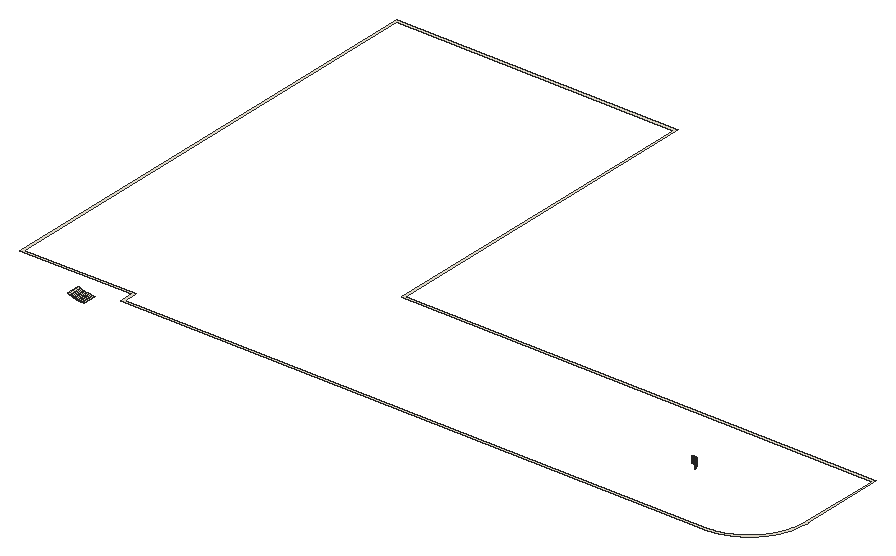
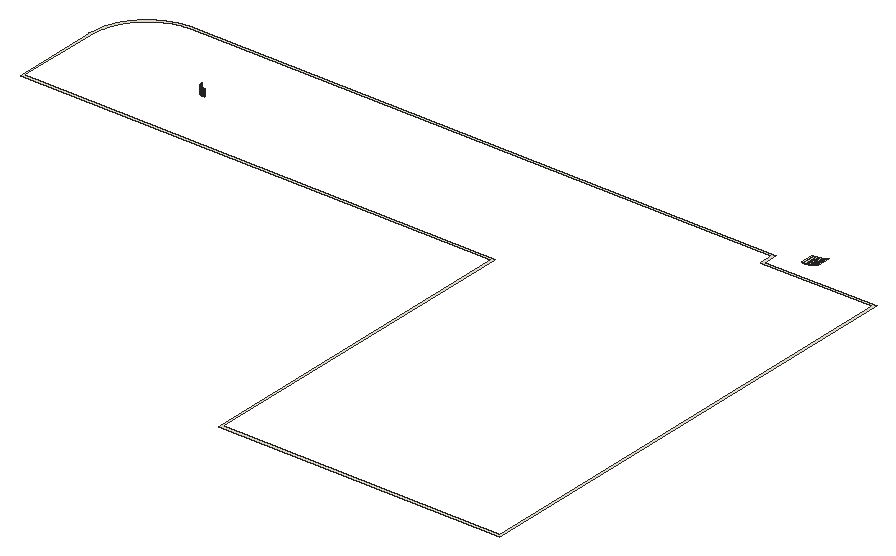
# SketchUp Ruby script. Lengths in inches.
U = 1.inch
M = Sketchup.active_model
def pt(a) = Geom::Point3d.new(a.map { |v| v * U })
def face(e, loops, mat)
  f = e.add_face(loops[0].map { |a| pt(a) })
  loops[1..].each { |l| e.add_face(l.map { |a| pt(a) }).erase! }
  f.material = f.back_material = mat if mat
  f
end
# faces: each face lists its corners as indices into pts; further lists are holes
def faces(e, pts, list, mat = nil) = list.each { |f| face(e, (f[0].is_a?(Array) ? f : [f]).map { |l| l.map { |i| pts[i] } }, mat) }
# xy, xz, yz: faces in a plane at the given z, y or x. An outline is a flat list of corners, or four numbers for a rectangle; further outlines are holes
def ring(l) = l.size == 4 ? [[l[0], l[1]], [l[2], l[1]], [l[2], l[3]], [l[0], l[3]]] : l.each_slice(2).to_a
def flat(e, list, mat, &to3) = list.each { |f| face(e, (f[0].is_a?(Array) ? f : [f]).map { |l| ring(l).map { |u, v| to3.(u, v) } }, mat) }
def xy(e, z, list, mat = nil) = flat(e, list, mat) { |x, y| [x, y, z] }
def xz(e, y, list, mat = nil) = flat(e, list, mat) { |x, z| [x, y, z] }
def yz(e, x, list, mat = nil) = flat(e, list, mat) { |y, z| [x, y, z] }
def lines(e, pts, list) = list.each { |a, b| e.add_line(pt(pts[a]), pt(pts[b])) }
# prism: a flat outline (further loops are holes) pulled along v
def prism(e, loops, v, mat = nil)
  f = face(e, loops, mat); d = Geom::Vector3d.new(v.map { |x| x * U })
  f.pushpull(f.normal.samedirection?(d) ? d.length : -d.length)
end
def box(e, o, s, mat = nil) = prism(e, [[o, [o[0] + s[0], o[1], o[2]], [o[0] + s[0], o[1] + s[1], o[2]], [o[0], o[1] + s[1], o[2]]]], [0, 0, s[2]], mat)
def at(x, y, z, deg = 0) = Geom::Transformation.translation(pt([x, y, z])) * Geom::Transformation.rotation(ORIGIN, Z_AXIS, deg.degrees)
def axes(o, x, y, z) = Geom::Transformation.new([*x, 0, *y, 0, *z, 0, *pt(o).to_a, 1])
def part(name) = M.definitions.add(name)
# library, detail: a bought-in or finely detailed component or shape, given as its bounding box
def library(name, o, s) = part(name).tap { |d| box(d.entities, o, s) }
def detail(e, o, s) = box(e.add_group.entities, o, s)
def put(e, d, t, mat = nil) = e.add_instance(d, t).tap { |i| i.material = mat if mat }
def group(e, t, mat = nil) = e.add_group.tap { |g| g.transformation = t; g.material = mat if mat }.entities
root = M.entities
M.materials.add("0027 AP L140 CRUSHED ICE").color = [241, 233, 217]
xy(root,120.5,[[[78,225,78,231,27,231,27,447,156,447,156,291,372,291,372,251.72,371.99,251.43,371.99,251.15,371.98,250.87,371.96,250.59,371.95,250.3,371.91,249.74,371.79,248.62,371.67,247.78,371.47,246.66,371.41,246.39,371.29,245.83,371.15,245.29,371.08,245.01,371.01,244.74,370.85,244.2,370.76,243.93,370.68,243.66,370.5,243.12,370.4,242.85,370.31,242.59,370.21,242.32,370.1,242.0625,370,241.8,369.67,241.02,369.43,240.5,369.31,240.25,369.18,239.99,369.06,239.74,368.8,239.24,368.66,238.99,368.52,238.75,368.38,238.5,368.24,238.26,368.09,238.01,367.95,237.77,367.8,237.53,367.64,237.29,367.49,237.06,367.33,236.82,367.01,236.36,366.84,236.13,366.68,235.9,366.51,235.68,366.33,235.45,366.16,235.23,365.62,234.57,365.4375,234.36,365.25,234.14,365.06,233.93,364.875,233.72,364.68,233.52,364.49,233.3125,364.29,233.11,363.89,232.71,363.6875,232.51,363.48,232.32,363.28,232.125,363.07,231.94,362.86,231.75,362.64,231.5625,362.43,231.38,361.77,230.84,361.55,230.67,361.32,230.49,361.1,230.32,360.87,230.16,360.64,229.99,360.18,229.67,359.94,229.51,359.71,229.36,359.47,229.2,359.23,229.05,358.99,228.91,358.74,228.76,358.5,228.62,358.25,228.48,358.01,228.34,357.76,228.2,357.26,227.94,357.01,227.82,356.75,227.69,356.5,227.57,355.98,227.33,355.2,227,354.9375,226.9,354.68,226.79,354.41,226.69,354.15,226.6,353.88,226.5,353.34,226.32,353.07,226.24,352.8,226.15,352.26,225.99,351.99,225.92,351.71,225.85,351.17,225.71,350.61,225.59,350.34,225.53,349.22,225.33,348.38,225.21,347.26,225.09,346.7,225.05,346.41,225.04,346.13,225.02,345.85,225.01,345.57,225.01,345.28,225],[79,226,345.27,226,345.54,226.01,345.82,226.01,346.09,226.02,346.36,226.04,346.63,226.05,346.9,226.07,347.18,226.09,347.45,226.12,347.72,226.14,347.99,226.17,348.26,226.21,348.53,226.24,349.34,226.36,349.6,226.41,350.14,226.51,350.41,226.57,350.67,226.625,350.9375,226.6875,351.2,226.75,351.47,226.82,352.25,227.03,352.51,227.11,352.78,227.19,353.03,227.27,353.81,227.54,354.0625,227.63,354.32,227.73,354.82,227.93,355.08,228.03,355.58,228.25,355.82,228.36,356.07,228.47,356.32,228.59,356.5625,228.71,356.8,228.83,357.05,228.96,357.53,229.22,357.76,229.35,358,229.48,358.24,229.62,358.7,229.9,358.93,230.05,359.16,230.19,359.39,230.34,359.61,230.5,359.84,230.65,360.0625,230.81,360.28,230.97,360.5,231.125,360.72,231.29,360.9375,231.46,361.15,231.625,361.36,231.79,361.57,231.97,361.78,232.14,361.99,232.32,362.19,232.5,362.4,232.68,362.6,232.86,362.8,233.05,363,233.23,363.19,233.42,363.38,233.62,363.58,233.81,363.77,234,363.95,234.2,364.14,234.4,364.32,234.6,364.5,234.81,364.68,235.01,364.86,235.22,365.03,235.43,365.21,235.64,365.375,235.85,365.54,236.0625,365.71,236.28,365.875,236.5,366.03,236.72,366.19,236.9375,366.35,237.16,366.5,237.39,366.66,237.61,366.81,237.84,366.95,238.07,367.1,238.3,367.38,238.76,367.52,239,367.65,239.24,367.78,239.47,368.04,239.95,368.17,240.2,368.29,240.4375,368.41,240.68,368.53,240.93,368.64,241.18,368.75,241.42,368.97,241.92,369.07,242.18,369.27,242.68,369.37,242.9375,369.46,243.19,369.73,243.97,369.81,244.22,369.89,244.49,369.97,244.75,370.18,245.53,370.25,245.8,370.3125,246.0625,370.375,246.33,370.43,246.59,370.49,246.86,370.59,247.4,370.64,247.66,370.76,248.47,370.79,248.74,370.83,249.01,370.86,249.28,370.88,249.55,370.91,249.82,370.93,250.1,370.95,250.37,370.96,250.64,370.98,250.91,370.99,251.18,370.99,251.46,371,251.73,371,290,155,290,155,446,28,446,28,232,79,232]]],"0027 AP L140 CRUSHED ICE")
xz(root,261,[[311.84,120,311.92,123],[311.92,120,312,123],[312,120,312.08,123],[312.08,120,312.16,123]],"0027 AP L140 CRUSHED ICE")
yz(root,315,[[258,120,258.08,123],[258.08,120,258.16,123]],"0027 AP L140 CRUSHED ICE")
p = [[67.49,216,120.05],[66.99,216,120.08],[66.99,222,120.08],[67.49,222,120.05],[67.99,216,120.02],[67.99,222,120.02],
  [68.5,216,120.01],[68.5,222,120.01],[314.98,258.3125,120],[314.99,258.24,120],[314.99,258.24,123],[314.98,258.3125,123],
  [315,258.16,120],[315,258.16,123],[314.97,258.39,120],[314.97,258.39,123],[314.96,258.47,120],[314.96,258.47,123],
  [314.93,258.625,120],[314.95,258.55,120],[314.95,258.55,123],[314.93,258.625,123],[314.92,258.7,120],[314.92,258.7,123],
  [314.9,258.78,120],[314.9,258.78,123],[314.875,258.85,120],[314.875,258.85,123],[314.83,259,120],[314.85,258.93,120],
  [314.85,258.93,123],[314.83,259,123],[314.8,259.08,120],[314.8,259.08,123],[314.74,259.22,120],[314.77,259.15,120],
  [314.77,259.15,123],[314.74,259.22,123],[314.71,259.29,120],[314.71,259.29,123],[314.67,259.36,120],[314.67,259.36,123],
  [314.6,259.5,120],[314.64,259.43,120],[314.64,259.43,123],[314.6,259.5,123],[314.56,259.57,120],[314.56,259.57,123],
  [314.47,259.7,120],[314.52,259.63,120],[314.52,259.63,123],[314.47,259.7,123],[314.43,259.76,120],[314.43,259.76,123],
  [314.33,259.89,120],[314.38,259.83,120],[314.38,259.83,123],[314.33,259.89,123],[314.23,260.01,120],[314.28,259.95,120],
  [314.28,259.95,123],[314.23,260.01,123],[314.18,260.07,120],[314.18,260.07,123],[314.07,260.18,120],[314.12,260.12,120],
  [314.12,260.12,123],[314.07,260.18,123],[313.95,260.28,120],[314.01,260.23,120],[314.01,260.23,123],[313.95,260.28,123],
  [313.83,260.38,120],[313.89,260.33,120],[313.89,260.33,123],[313.83,260.38,123],[313.7,260.47,120],[313.76,260.43,120],
  [313.76,260.43,123],[313.7,260.47,123],[313.57,260.56,120],[313.63,260.52,120],[313.63,260.52,123],[313.57,260.56,123],
  [313.36,260.67,120],[313.43,260.64,120],[313.43,260.64,123],[313.36,260.67,123],[313.5,260.6,120],[313.5,260.6,123],
  [313.15,260.77,120],[313.22,260.74,120],[313.22,260.74,123],[313.15,260.77,123],[313.29,260.71,120],[313.29,260.71,123],
  [312.93,260.85,120],[313,260.83,120],[313,260.83,123],[312.93,260.85,123],[313.08,260.8,120],[313.08,260.8,123],
  [311.3,260.92,120],[311.375,260.93,120],[311.375,260.93,123],[311.3,260.92,123],[311.45,260.95,120],[311.45,260.95,123],
  [311.53,260.96,120],[311.53,260.96,123],[312.47,260.96,120],[312.55,260.95,120],[312.55,260.95,123],[312.47,260.96,123],
  [312.625,260.93,120],[312.625,260.93,123],[312.7,260.92,120],[312.7,260.92,123],[312.78,260.9,120],[312.78,260.9,123],
  [312.85,260.875,120],[312.85,260.875,123],[311.61,260.97,120],[311.61,260.97,123],[311.6875,260.98,120],[311.6875,260.98,123],
  [311.76,260.99,120],[311.76,260.99,123],[311.84,261,120],[311.84,261,123],[312.16,261,120],[312.24,260.99,120],
  [312.24,260.99,123],[312.16,261,123],[312.3125,260.98,120],[312.3125,260.98,123],[312.39,260.97,120],[312.39,260.97,123],
  [66.49,216,120.13],[65.99,216,120.1875],[65.99,222,120.1875],[66.49,222,120.13],[65.49,216,120.26],[65.49,222,120.26],
  [65,216,120.34],[64.5,216,120.43],[64.5,222,120.43],[65,222,120.34],[64.01,216,120.52],[64.01,222,120.52],
  [63.52,216,120.63],[63.52,222,120.63],[63.03,216,120.75],[63.03,222,120.75],[62.55,216,120.88],[62.55,222,120.88],
  [62.0625,216,121.02],[62.0625,222,121.02],[61.58,216,121.17],[61.58,222,121.17],[61.11,216,121.34],[61.11,222,121.34],
  [60.63,216,121.51],[60.63,222,121.51]]
faces(root,p,[[0,1,2,3],[4,0,3,5],[6,4,5,7],[8,9,10,11],[9,12,13,10],[14,8,11,15],[16,14,15,17],[18,19,20,21],
  [19,16,17,20],[22,18,21,23],[24,22,23,25],[26,24,25,27],[28,29,30,31],[29,26,27,30],[32,28,31,33],[34,35,36,37],
  [35,32,33,36],[38,34,37,39],[40,38,39,41],[42,43,44,45],[43,40,41,44],[46,42,45,47],[48,49,50,51],[49,46,47,50],
  [52,48,51,53],[54,55,56,57],[55,52,53,56],[58,59,60,61],[59,54,57,60],[62,58,61,63],[64,65,66,67],[65,62,63,66],
  [68,69,70,71],[69,64,67,70],[72,73,74,75],[73,68,71,74],[76,77,78,79],[77,72,75,78],[80,81,82,83],[81,76,79,82],
  [84,85,86,87],[85,88,89,86],[88,80,83,89],[90,91,92,93],[91,94,95,92],[94,84,87,95],[96,97,98,99],[97,100,101,98],
  [100,90,93,101],[102,103,104,105],[103,106,107,104],[106,108,109,107],[110,111,112,113],[111,114,115,112],[114,116,117,115],[116,118,119,117],
  [118,120,121,119],[120,96,99,121],[108,122,123,109],[122,124,125,123],[124,126,127,125],[126,128,129,127],[130,131,132,133],[131,134,135,132],
  [134,136,137,135],[136,110,113,137],[138,139,140,141],[1,138,141,2],[139,142,143,140],[144,145,146,147],[142,144,147,143],[145,148,149,146],
  [148,150,151,149],[150,152,153,151],[152,154,155,153],[154,156,157,155],[156,158,159,157],[158,160,161,159],[160,162,163,161]],"0027 AP L140 CRUSHED ICE")
